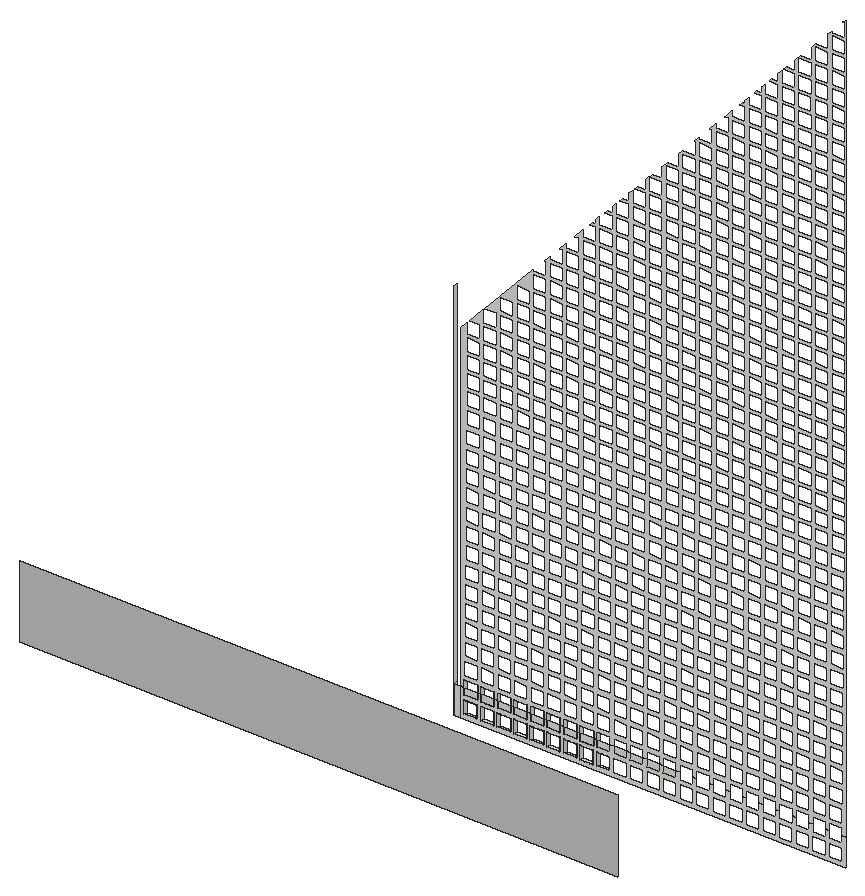
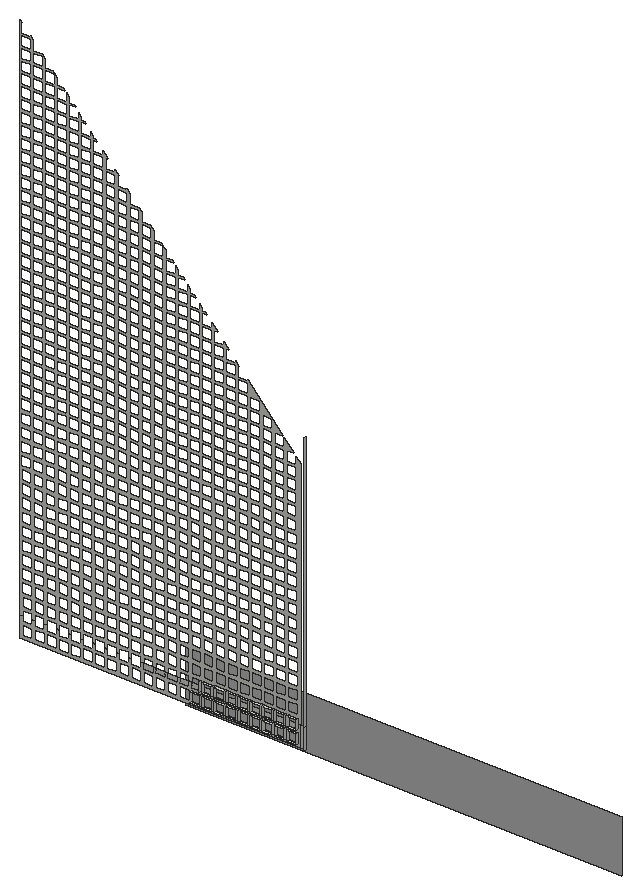
# SketchUp Ruby script. Lengths in inches.
U = 1.inch
M = Sketchup.active_model
def pt(a) = Geom::Point3d.new(a.map { |v| v * U })
def face(e, loops, mat)
  f = e.add_face(loops[0].map { |a| pt(a) })
  loops[1..].each { |l| e.add_face(l.map { |a| pt(a) }).erase! }
  f.material = f.back_material = mat if mat
  f
end
# faces: each face lists its corners as indices into pts; further lists are holes
def faces(e, pts, list, mat = nil) = list.each { |f| face(e, (f[0].is_a?(Array) ? f : [f]).map { |l| l.map { |i| pts[i] } }, mat) }
# xy, xz, yz: faces in a plane at the given z, y or x. An outline is a flat list of corners, or four numbers for a rectangle; further outlines are holes
def ring(l) = l.size == 4 ? [[l[0], l[1]], [l[2], l[1]], [l[2], l[3]], [l[0], l[3]]] : l.each_slice(2).to_a
def flat(e, list, mat, &to3) = list.each { |f| face(e, (f[0].is_a?(Array) ? f : [f]).map { |l| ring(l).map { |u, v| to3.(u, v) } }, mat) }
def xy(e, z, list, mat = nil) = flat(e, list, mat) { |x, y| [x, y, z] }
def xz(e, y, list, mat = nil) = flat(e, list, mat) { |x, z| [x, y, z] }
def yz(e, x, list, mat = nil) = flat(e, list, mat) { |y, z| [x, y, z] }
def lines(e, pts, list) = list.each { |a, b| e.add_line(pt(pts[a]), pt(pts[b])) }
# prism: a flat outline (further loops are holes) pulled along v
def prism(e, loops, v, mat = nil)
  f = face(e, loops, mat); d = Geom::Vector3d.new(v.map { |x| x * U })
  f.pushpull(f.normal.samedirection?(d) ? d.length : -d.length)
end
def box(e, o, s, mat = nil) = prism(e, [[o, [o[0] + s[0], o[1], o[2]], [o[0] + s[0], o[1] + s[1], o[2]], [o[0], o[1] + s[1], o[2]]]], [0, 0, s[2]], mat)
def at(x, y, z, deg = 0) = Geom::Transformation.translation(pt([x, y, z])) * Geom::Transformation.rotation(ORIGIN, Z_AXIS, deg.degrees)
def axes(o, x, y, z) = Geom::Transformation.new([*x, 0, *y, 0, *z, 0, *pt(o).to_a, 1])
def part(name) = M.definitions.add(name)
# library, detail: a bought-in or finely detailed component or shape, given as its bounding box
def library(name, o, s) = part(name).tap { |d| box(d.entities, o, s) }
def detail(e, o, s) = box(e.add_group.entities, o, s)
def put(e, d, t, mat = nil) = e.add_instance(d, t).tap { |i| i.material = mat if mat }
def group(e, t, mat = nil) = e.add_group.tap { |g| g.transformation = t; g.material = mat if mat }.entities
root = M.entities
M.materials.add("[Color M02]").color = [198, 198, 198]
xy(root,259.68,[[432.73,480.14,435.05,480.77],[435.65,480.14,437.96,480.77],[438.56,480.14,440.87,480.77],[441.47,480.14,443.78,480.77],[444.38,480.14,446.69,480.77],
  [447.29,480.14,449.61,480.77],[450.21,480.14,452.52,480.77],[453.12,480.14,455.43,480.77],[456.03,480.14,458.34,480.77]])
xy(root,262,[[432.73,480.14,435.05,480.77],[435.65,480.14,437.96,480.77],[438.56,480.14,440.87,480.77],[441.47,480.14,443.78,480.77],[444.38,480.14,446.69,480.77],
  [447.29,480.14,449.61,480.77],[450.21,480.14,452.52,480.77],[453.12,480.14,455.43,480.77],[456.03,480.14,458.34,480.77]])
xy(root,262.73,[[432.76,480.14,435.08,480.77],[435.68,480.14,437.99,480.77],[438.59,480.14,440.9,480.77],[441.5,480.14,443.8125,480.77],[444.41,480.14,446.72,480.77],
  [447.32,480.14,449.64,480.77],[450.24,480.14,452.55,480.77],[453.15,480.14,455.46,480.77]])
xy(root,265.04,[[432.76,480.14,435.08,480.77],[435.68,480.14,437.99,480.77],[438.59,480.14,440.9,480.77],[441.5,480.14,443.8125,480.77],[444.41,480.14,446.72,480.77],
  [447.32,480.14,449.64,480.77],[450.24,480.14,452.55,480.77],[453.15,480.14,455.46,480.77]])
xz(root,469.875,[[363.02,251.0625,468.02,263.89]],"[Color M02]")
xz(root,480.14,[[430.97,258.95,432.11,263.89],[[432.11,258.95,499.71,258.95,499.71,263.89,499.14,263.89,499.14,262.73,496.83,262.73,496.83,263.89,496.23,263.89,496.23,262.73,493.92,262.73,493.92,263.89,493.32,263.89,493.32,262.73,491,262.73,491,263.89,490.4,263.89,490.4,262.73,488.09,262.73,488.09,263.89,487.49,263.89,487.49,262.73,485.18,262.73,485.18,263.89,484.58,263.89,484.58,262.73,482.27,262.73,482.27,263.89,481.67,263.89,481.67,262.73,479.36,262.73,479.36,263.89,478.76,263.89,478.76,262.73,476.44,262.73,476.44,263.89,475.84,263.89,475.84,262.73,473.53,262.73,473.53,263.89,472.93,263.89,472.93,262.73,470.62,262.73,470.62,263.89,470.02,263.89,470.02,262.73,467.71,262.73,467.71,263.89,467.11,263.89,467.11,262.73,464.8,262.73,464.8,263.89,464.2,263.89,464.2,262.73,461.88,262.73,461.88,263.89,461.28,263.89,461.28,262.73,458.97,262.73,458.97,263.89,458.37,263.89,458.37,262.73,456.06,262.73,456.06,263.89,455.46,263.89,455.46,262.73,453.15,262.73,453.15,263.89,452.55,263.89,452.55,262.73,450.24,262.73,450.24,263.89,449.64,263.89,449.64,262.73,447.32,262.73,447.32,263.89,446.72,263.89,446.72,262.73,444.41,262.73,444.41,263.89,443.8125,263.89,443.8125,262.73,441.5,262.73,441.5,263.89,440.9,263.89,440.9,262.73,438.59,262.73,438.59,263.89,437.99,263.89,437.99,262.73,435.68,262.73,435.68,263.89,435.08,263.89,435.08,262.73,432.76,262.73,432.76,263.89,432.11,263.89],[496.8,259.68,499.11,262],[493.89,259.68,496.2,262],[490.97,259.68,493.29,262],[488.0625,259.68,490.375,262],[485.15,259.68,487.46,262],[482.24,259.68,484.55,262],[479.33,259.68,481.64,262],[476.41,259.68,478.73,262],[473.5,259.68,475.81,262],[470.59,259.68,472.9,262],[467.68,259.68,469.99,262],[464.77,259.68,467.08,262],[461.85,259.68,464.17,262],[458.94,259.68,461.25,262],[456.03,259.68,458.34,262],[453.12,259.68,455.43,262],[450.21,259.68,452.52,262],[447.29,259.68,449.61,262],[444.38,259.68,446.69,262],[441.47,259.68,443.78,262],[438.56,259.68,440.87,262],[435.65,259.68,437.96,262],[432.73,259.68,435.05,262]],[432.76,262.73,435.08,263.89],[435.68,262.73,437.99,263.89],[438.59,262.73,440.9,263.89],
  [441.5,262.73,443.8125,263.89],[444.41,262.73,446.72,263.89],[447.32,262.73,449.64,263.89],[450.24,262.73,452.55,263.89],[453.15,262.73,455.46,263.89],
  [456.06,262.73,458.37,263.89],[458.97,262.73,461.28,263.89],[461.88,262.73,464.2,263.89],[464.8,262.73,467.11,263.89],[467.71,262.73,470.02,263.89],
  [[432.11,263.89,432.76,263.89,432.76,265.04,435.08,265.04,435.08,263.89,435.68,263.89,435.68,265.04,437.99,265.04,437.99,263.89,438.59,263.89,438.59,265.04,440.9,265.04,440.9,263.89,441.5,263.89,441.5,265.04,443.8125,265.04,443.8125,263.89,444.41,263.89,444.41,265.04,446.72,265.04,446.72,263.89,447.32,263.89,447.32,265.04,449.64,265.04,449.64,263.89,450.24,263.89,450.24,265.04,452.55,265.04,452.55,263.89,453.15,263.89,453.15,265.04,455.46,265.04,455.46,263.89,456.06,263.89,456.06,265.04,458.37,265.04,458.37,263.89,458.97,263.89,458.97,265.04,461.28,265.04,461.28,263.89,461.88,263.89,461.88,265.04,464.2,265.04,464.2,263.89,464.8,263.89,464.8,265.04,467.11,265.04,467.11,263.89,467.71,263.89,467.71,265.04,470.02,265.04,470.02,263.89,470.62,263.89,470.62,265.04,472.93,265.04,472.93,263.89,473.53,263.89,473.53,265.04,475.84,265.04,475.84,263.89,476.44,263.89,476.44,265.04,478.76,265.04,478.76,263.89,479.36,263.89,479.36,265.04,481.67,265.04,481.67,263.89,482.27,263.89,482.27,265.04,484.58,265.04,484.58,263.89,485.18,263.89,485.18,265.04,487.49,265.04,487.49,263.89,488.09,263.89,488.09,265.04,490.4,265.04,490.4,263.89,491,263.89,491,265.04,493.32,265.04,493.32,263.89,493.92,263.89,493.92,265.04,496.23,265.04,496.23,263.89,496.83,263.89,496.83,265.04,499.14,265.04,499.14,263.89,499.71,263.89,499.71,392.36,499.28,391.9,499.58,391.9,499.58,389.59,497.26,389.59,497.26,389.75,496.66,389.11,496.66,386.84,494.54,386.84,493.75,386,493.75,384.09,491.96,384.09,491.64,383.75,491.55,383.65,493.75,383.65,493.75,381.34,491.4375,381.34,491.4375,383.53,490.84,382.89,490.84,381.34,489.38,381.34,488.97,380.9,490.84,380.9,490.84,378.59,488.53,378.59,488.53,380.43,487.93,379.79,487.93,378.59,486.8,378.59,486.39,378.15,487.93,378.15,487.93,375.84,485.61,375.84,485.61,377.32,485.02,376.68,485.02,375.84,484.23,375.84,483.82,375.4,485.02,375.4,485.02,373.09,482.7,373.09,482.7,374.21,482.1,373.57,482.1,373.09,481.65,373.09,481.18,372.59,482.1,372.59,482.1,370.27,479.79,370.27,479.79,371.11,479.19,370.47,479.19,370.27,479.01,370.27,478.54,369.77,479.19,369.77,479.19,367.46,476.88,367.46,476.88,368,475.91,366.96,476.28,366.96,476.28,364.65,473.97,364.65,473.97,364.89,473.27,364.15,473.37,364.15,473.37,361.84,471.1,361.84,470.45,361.14,470.45,359.02,468.47,359.02,467.54,358.04,467.54,356.21,465.83,356.21,465.36,355.71,467.54,355.71,467.54,353.4,465.23,353.4,465.23,355.57,464.63,354.93,464.63,353.4,463.19,353.4,462.73,352.9,464.63,352.9,464.63,350.59,462.32,350.59,462.32,352.46,461.72,351.82,461.72,350.59,460.56,350.59,460.09,350.09,461.72,350.09,461.72,347.77,459.41,347.77,459.41,349.36,458.81,348.72,458.81,347.77,457.92,347.77,457.45,347.27,458.81,347.27,458.81,344.96,456.49,344.96,456.49,346.25,455.89,345.61,455.89,344.96,455.29,344.96,454.82,344.46,455.89,344.46,455.89,342.15,453.58,342.15,453.58,343.14,452.18,341.65,452.98,341.65,452.98,339.34,450.67,339.34,450.67,340.04,449.55,338.84,450.07,338.84,450.07,336.52,447.76,336.52,447.76,336.93,446.91,336.02,447.16,336.02,447.16,333.71,444.85,333.71,444.85,333.82,436.37,324.77,438.42,324.77,438.42,322.46,436.11,322.46,436.11,324.5,433.73,321.96,435.51,321.96,435.51,319.65,433.2,319.65,433.2,321.39,432.11,320.24],[497.26,375.84,499.58,378.15],[494.33,373.09,496.64,375.4],[497.26,373.09,499.58,375.4],[494.33,370.27,496.64,372.59],[497.26,370.27,499.58,372.59],[485.59,370.27,487.9,372.59],[488.53,370.27,490.84,372.59],[488.5,373.09,490.8125,375.4],[491.4375,373.09,493.75,375.4],[491.41,375.84,493.73,378.15],[494.35,375.84,496.66,378.15],[494.33,378.59,496.64,380.9],[497.26,378.59,499.58,380.9],[494.33,381.34,496.64,383.65],[497.26,381.34,499.58,383.65],[465.23,350.59,467.54,352.9],[462.32,347.77,464.63,350.09],[465.23,347.77,467.54,350.09],[459.41,344.96,461.72,347.27],[462.32,344.96,464.63,347.27],[465.23,344.96,467.54,347.27],[468.14,344.96,470.45,347.27],[471.05,344.96,473.37,347.27],[473.97,344.96,476.28,347.27],[476.88,344.96,479.19,347.27],[479.79,344.96,482.1,347.27],[482.7,344.96,485.02,347.27],[485.61,344.96,487.93,347.27],[488.53,344.96,490.84,347.27],[491.4375,344.96,493.75,347.27],[494.35,344.96,496.66,347.27],[497.26,344.96,499.58,347.27],[468.14,347.77,470.45,350.09],[471.05,347.77,473.37,350.09],[473.97,347.77,476.28,350.09],[476.88,347.77,479.19,350.09],[479.79,347.77,482.1,350.09],[482.7,347.77,485.02,350.09],[485.61,347.77,487.93,350.09],[488.53,347.77,490.84,350.09],[491.4375,347.77,493.75,350.09],[494.35,347.77,496.66,350.09],[497.26,347.77,499.58,350.09],[468.14,350.59,470.45,352.9],[471.05,350.59,473.37,352.9],[473.97,350.59,476.28,352.9],[476.88,350.59,479.19,352.9],[479.79,350.59,482.1,352.9],[482.7,350.59,485.02,352.9],[485.61,350.59,487.93,352.9],[488.53,350.59,490.84,352.9],[491.4375,350.59,493.75,352.9],[494.35,350.59,496.66,352.9],[497.26,350.59,499.58,352.9],[468.14,353.4,470.45,355.71],[471.05,353.4,473.37,355.71],[473.97,353.4,476.28,355.71],[476.88,353.4,479.19,355.71],[479.79,353.4,482.1,355.71],[482.7,353.4,485.02,355.71],[485.61,353.4,487.93,355.71],[488.53,353.4,490.84,355.71],[491.4375,353.4,493.75,355.71],[494.35,353.4,496.66,355.71],[497.26,353.4,499.58,355.71],[479.79,367.46,482.1,369.77],[482.7,367.46,485.02,369.77],[491.4375,367.46,493.75,369.77],[497.26,367.46,499.58,369.77],[488.53,367.46,490.84,369.77],[485.61,367.46,487.93,369.77],[494.35,367.46,496.66,369.77],[479.79,364.65,482.1,366.96],[485.61,364.65,487.93,366.96],[494.35,364.65,496.66,366.96],[491.4375,364.65,493.75,366.96],[482.7,364.65,485.02,366.96],[488.53,364.65,490.84,366.96],[497.26,364.65,499.58,366.96],[476.88,364.65,479.19,366.96],[488.53,361.84,490.84,364.15],[494.35,361.84,496.66,364.15],[482.7,361.84,485.02,364.15],[485.61,361.84,487.93,364.15],[497.26,361.84,499.58,364.15],[476.88,361.84,479.19,364.15],[473.97,361.84,476.28,364.15],[479.79,361.84,482.1,364.15],[491.4375,361.84,493.75,364.15],[488.53,359.02,490.84,361.34],[494.35,359.02,496.66,361.34],[482.7,359.02,485.02,361.34],[471.05,359.02,473.37,361.34],[497.26,359.02,499.58,361.34],[485.61,359.02,487.93,361.34],[476.88,359.02,479.19,361.34],[473.97,359.02,476.28,361.34],[491.4375,359.02,493.75,361.34],[479.79,359.02,482.1,361.34],[491.4375,356.21,493.75,358.52],[479.79,356.21,482.1,358.52],[473.97,356.21,476.28,358.52],[485.61,356.21,487.93,358.52],[497.26,356.21,499.58,358.52],[468.14,356.21,470.45,358.52],[476.88,356.21,479.19,358.52],[471.05,356.21,473.37,358.52],[482.7,356.21,485.02,358.52],[494.35,356.21,496.66,358.52],[488.53,356.21,490.84,358.52],[456.49,342.15,458.81,344.46],[459.41,342.15,461.72,344.46],[462.32,342.15,464.63,344.46],[465.23,342.15,467.54,344.46],[468.14,342.15,470.45,344.46],[471.05,342.15,473.37,344.46],[473.97,342.15,476.28,344.46],[476.88,342.15,479.19,344.46],[479.79,342.15,482.1,344.46],[482.7,342.15,485.02,344.46],[485.61,342.15,487.93,344.46],[488.53,342.15,490.84,344.46],[491.4375,342.15,493.75,344.46],[494.35,342.15,496.66,344.46],[497.26,342.15,499.58,344.46],[453.58,339.34,455.89,341.65],[456.49,339.34,458.81,341.65],[459.41,339.34,461.72,341.65],[462.32,339.34,464.63,341.65],[465.23,339.34,467.54,341.65],[468.14,339.34,470.45,341.65],[471.05,339.34,473.37,341.65],[473.97,339.34,476.28,341.65],[476.88,339.34,479.19,341.65],[479.79,339.34,482.1,341.65],[482.7,339.34,485.02,341.65],[485.61,339.34,487.93,341.65],[488.53,339.34,490.84,341.65],[491.4375,339.34,493.75,341.65],[494.35,339.34,496.66,341.65],[497.26,339.34,499.58,341.65],[450.67,336.52,452.98,338.84],[453.58,336.52,455.89,338.84],[456.49,336.52,458.81,338.84],[459.41,336.52,461.72,338.84],[462.32,336.52,464.63,338.84],[465.23,336.52,467.54,338.84],[468.14,336.52,470.45,338.84],[471.05,336.52,473.37,338.84],[473.97,336.52,476.28,338.84],[476.88,336.52,479.19,338.84],[479.79,336.52,482.1,338.84],[482.7,336.52,485.02,338.84],[485.61,336.52,487.93,338.84],[488.53,336.52,490.84,338.84],[491.4375,336.52,493.75,338.84],[494.35,336.52,496.66,338.84],[497.26,336.52,499.58,338.84],[447.76,333.71,450.07,336.02],[450.67,333.71,452.98,336.02],[453.58,333.71,455.89,336.02],[456.49,333.71,458.81,336.02],[459.41,333.71,461.72,336.02],[462.32,333.71,464.63,336.02],[465.23,333.71,467.54,336.02],[468.14,333.71,470.45,336.02],[471.05,333.71,473.37,336.02],[473.97,333.71,476.28,336.02],[476.88,333.71,479.19,336.02],[479.79,333.71,482.1,336.02],[482.7,333.71,485.02,336.02],[485.61,333.71,487.93,336.02],[488.53,333.71,490.84,336.02],[491.4375,333.71,493.75,336.02],[494.35,333.71,496.66,336.02],[497.26,333.71,499.58,336.02],[444.85,330.9,447.16,333.21],[447.76,330.9,450.07,333.21],[450.67,330.9,452.98,333.21],[453.58,330.9,455.89,333.21],[456.49,330.9,458.81,333.21],[459.41,330.9,461.72,333.21],[462.32,330.9,464.63,333.21],[465.23,330.9,467.54,333.21],[468.14,330.9,470.45,333.21],[471.05,330.9,473.37,333.21],[473.97,330.9,476.28,333.21],[476.88,330.9,479.19,333.21],[479.79,330.9,482.1,333.21],[482.7,330.9,485.02,333.21],[485.61,330.9,487.93,333.21],[488.53,330.9,490.84,333.21],[491.4375,330.9,493.75,333.21],[494.35,330.9,496.66,333.21],[497.26,330.9,499.58,333.21],[441.93,328.09,444.25,330.4],[444.85,328.09,447.16,330.4],[447.76,328.09,450.07,330.4],[450.67,328.09,452.98,330.4],[453.58,328.09,455.89,330.4],[456.49,328.09,458.81,330.4],[459.41,328.09,461.72,330.4],[462.32,328.09,464.63,330.4],[465.23,328.09,467.54,330.4],[468.14,328.09,470.45,330.4],[471.05,328.09,473.37,330.4],[473.97,328.09,476.28,330.4],[476.88,328.09,479.19,330.4],[479.79,328.09,482.1,330.4],[482.7,328.09,485.02,330.4],[485.61,328.09,487.93,330.4],[488.53,328.09,490.84,330.4],[491.4375,328.09,493.75,330.4],[494.35,328.09,496.66,330.4],[497.26,328.09,499.58,330.4],[439.02,325.27,441.33,327.59],[441.93,325.27,444.25,327.59],[444.85,325.27,447.16,327.59],[447.76,325.27,450.07,327.59],[450.67,325.27,452.98,327.59],[453.58,325.27,455.89,327.59],[456.49,325.27,458.81,327.59],[459.41,325.27,461.72,327.59],[462.32,325.27,464.63,327.59],[465.23,325.27,467.54,327.59],[468.14,325.27,470.45,327.59],[471.05,325.27,473.37,327.59],[473.97,325.27,476.28,327.59],[476.88,325.27,479.19,327.59],[479.79,325.27,482.1,327.59],[482.7,325.27,485.02,327.59],[485.61,325.27,487.93,327.59],[488.53,325.27,490.84,327.59],[491.4375,325.27,493.75,327.59],[494.35,325.27,496.66,327.59],[497.26,325.27,499.58,327.59],[439.02,322.46,441.33,324.77],[441.93,322.46,444.25,324.77],[444.85,322.46,447.16,324.77],[447.76,322.46,450.07,324.77],[450.67,322.46,452.98,324.77],[453.58,322.46,455.89,324.77],[456.49,322.46,458.81,324.77],[459.41,322.46,461.72,324.77],[462.32,322.46,464.63,324.77],[465.23,322.46,467.54,324.77],[468.14,322.46,470.45,324.77],[471.05,322.46,473.37,324.77],[473.97,322.46,476.28,324.77],[476.88,322.46,479.19,324.77],[479.79,322.46,482.1,324.77],[482.7,322.46,485.02,324.77],[485.61,322.46,487.93,324.77],[488.53,322.46,490.84,324.77],[491.4375,322.46,493.75,324.77],[494.35,322.46,496.66,324.77],[497.26,322.46,499.58,324.77],[436.11,319.65,438.42,321.96],[439.02,319.65,441.33,321.96],[441.93,319.65,444.25,321.96],[444.85,319.65,447.16,321.96],[447.76,319.65,450.07,321.96],[450.67,319.65,452.98,321.96],[453.58,319.65,455.89,321.96],[456.49,319.65,458.81,321.96],[459.41,319.65,461.72,321.96],[462.32,319.65,464.63,321.96],[465.23,319.65,467.54,321.96],[468.14,319.65,470.45,321.96],[471.05,319.65,473.37,321.96],[473.97,319.65,476.28,321.96],[476.88,319.65,479.19,321.96],[479.79,319.65,482.1,321.96],[482.7,319.65,485.02,321.96],[485.61,319.65,487.93,321.96],[488.53,319.65,490.84,321.96],[491.4375,319.65,493.75,321.96],[494.35,319.65,496.66,321.96],[497.26,319.65,499.58,321.96],[433.2,316.84,435.51,319.15],[436.11,316.84,438.42,319.15],[439.02,316.84,441.33,319.15],[441.93,316.84,444.25,319.15],[444.85,316.84,447.16,319.15],[447.76,316.84,450.07,319.15],[450.67,316.84,452.98,319.15],[453.58,316.84,455.89,319.15],[456.49,316.84,458.81,319.15],[459.41,316.84,461.72,319.15],[462.32,316.84,464.63,319.15],[465.23,316.84,467.54,319.15],[468.14,316.84,470.45,319.15],[471.05,316.84,473.37,319.15],[473.97,316.84,476.28,319.15],[476.88,316.84,479.19,319.15],[479.79,316.84,482.1,319.15],[482.7,316.84,485.02,319.15],[485.61,316.84,487.93,319.15],[488.53,316.84,490.84,319.15],[491.4375,316.84,493.75,319.15],[494.35,316.84,496.66,319.15],[497.26,316.84,499.58,319.15],[433.2,314.02,435.51,316.34],[436.11,314.02,438.42,316.34],[439.02,314.02,441.33,316.34],[441.93,314.02,444.25,316.34],[444.85,314.02,447.16,316.34],[447.76,314.02,450.07,316.34],[450.67,314.02,452.98,316.34],[453.58,314.02,455.89,316.34],[456.49,314.02,458.81,316.34],[459.41,314.02,461.72,316.34],[462.32,314.02,464.63,316.34],[465.23,314.02,467.54,316.34],[468.14,314.02,470.45,316.34],[471.05,314.02,473.37,316.34],[473.97,314.02,476.28,316.34],[476.88,314.02,479.19,316.34],[479.79,314.02,482.1,316.34],[482.7,314.02,485.02,316.34],[485.61,314.02,487.93,316.34],[488.53,314.02,490.84,316.34],[491.4375,314.02,493.75,316.34],[494.35,314.02,496.66,316.34],[497.26,314.02,499.58,316.34],[450.67,311.21,452.98,313.52],[453.58,311.21,455.89,313.52],[439.02,311.21,441.33,313.52],[433.2,311.21,435.51,313.52],[494.35,311.21,496.66,313.52],[476.88,311.21,479.19,313.52],[465.23,311.21,467.54,313.52],[441.93,311.21,444.25,313.52],[471.05,311.21,473.37,313.52],[468.14,311.21,470.45,313.52],[444.85,311.21,447.16,313.52],[482.7,311.21,485.02,313.52],[456.49,311.21,458.81,313.52],[491.4375,311.21,493.75,313.52],[485.61,311.21,487.93,313.52],[436.11,311.21,438.42,313.52],[479.79,311.21,482.1,313.52],[488.53,311.21,490.84,313.52],[462.32,311.21,464.63,313.52],[497.26,311.21,499.58,313.52],[447.76,311.21,450.07,313.52],[459.41,311.21,461.72,313.52],[473.97,311.21,476.28,313.52],[433.2,308.4,435.51,310.71],[436.11,308.4,438.42,310.71],[439.02,308.4,441.33,310.71],[441.93,308.4,444.25,310.71],[444.85,308.4,447.16,310.71],[447.76,308.4,450.07,310.71],[450.67,308.4,452.98,310.71],[453.58,308.4,455.89,310.71],[456.49,308.4,458.81,310.71],[459.41,308.4,461.72,310.71],[462.32,308.4,464.63,310.71],[465.23,308.4,467.54,310.71],[468.14,308.4,470.45,310.71],[471.05,308.4,473.37,310.71],[473.97,308.4,476.28,310.71],[476.88,308.4,479.19,310.71],[479.79,308.4,482.1,310.71],[482.7,308.4,485.02,310.71],[485.61,308.4,487.93,310.71],[488.53,308.4,490.84,310.71],[491.4375,308.4,493.75,310.71],[494.35,308.4,496.66,310.71],[497.26,308.4,499.58,310.71],[433.17,305.35,435.48,307.67],[436.08,305.35,438.39,307.67],[438.99,305.35,441.31,307.67],[441.91,305.35,444.22,307.67],[444.82,305.35,447.13,307.67],[447.73,305.35,450.04,307.67],[450.64,305.35,452.95,307.67],[453.55,305.35,455.87,307.67],[456.47,305.35,458.78,307.67],[459.38,305.35,461.69,307.67],[462.29,305.35,464.6,307.67],[465.2,305.35,467.51,307.67],[468.11,305.35,470.43,307.67],[471.03,305.35,473.34,307.67],[473.9375,305.35,476.25,307.67],[476.85,305.35,479.16,307.67],[479.76,305.35,482.07,307.67],[482.67,305.35,484.99,307.67],[485.59,305.35,487.9,307.67],[488.5,305.35,490.81,307.67],[491.41,305.35,493.72,307.67],[494.32,305.35,496.63,307.67],[497.23,305.35,499.55,307.67],[433.14,302.31,435.45,304.62],[436.05,302.31,438.36,304.62],[438.96,302.31,441.28,304.62],[441.875,302.31,444.1875,304.62],[444.79,302.31,447.1,304.62],[447.7,302.31,450.01,304.62],[450.61,302.31,452.92,304.62],[453.52,302.31,455.84,304.62],[456.4375,302.31,458.75,304.62],[459.35,302.31,461.66,304.62],[462.26,302.31,464.57,304.62],[465.17,302.31,467.48,304.62],[468.08,302.31,470.4,304.62],[471,302.31,473.31,304.62],[473.91,302.31,476.22,304.62],[476.82,302.31,479.13,304.62],[479.73,302.31,482.04,304.62],[482.64,302.31,484.96,304.62],[485.56,302.31,487.87,304.62],[488.47,302.31,490.78,304.62],[491.38,302.31,493.69,304.62],[494.29,302.31,496.61,304.62],[497.2,302.31,499.52,304.62],[433.11,299.27,435.42,301.58],[436.02,299.27,438.34,301.58],[438.93,299.27,441.25,301.58],[441.85,299.27,444.16,301.58],[444.76,299.27,447.07,301.58],[447.67,299.27,449.98,301.58],[450.58,299.27,452.9,301.58],[453.5,299.27,455.81,301.58],[456.41,299.27,458.72,301.58],[459.32,299.27,461.63,301.58],[462.23,299.27,464.54,301.58],[465.14,299.27,467.46,301.58],[468.06,299.27,470.37,301.58],[470.97,299.27,473.28,301.58],[473.88,299.27,476.19,301.58],[476.79,299.27,479.1,301.58],[479.7,299.27,482.02,301.58],[482.62,299.27,484.93,301.58],[485.53,299.27,487.84,301.58],[488.44,299.27,490.75,301.58],[491.35,299.27,493.66,301.58],[494.26,299.27,496.58,301.58],[497.18,299.27,499.49,301.58],[433.08,296.22,435.39,298.53],[435.99,296.22,438.31,298.53],[438.91,296.22,441.22,298.53],[441.82,296.22,444.13,298.53],[444.73,296.22,447.04,298.53],[447.64,296.22,449.95,298.53],[450.55,296.22,452.87,298.53],[453.47,296.22,455.78,298.53],[456.38,296.22,458.69,298.53],[459.29,296.22,461.6,298.53],[462.2,296.22,464.51,298.53],[465.11,296.22,467.43,298.53],[468.03,296.22,470.34,298.53],[470.9375,296.22,473.25,298.53],[473.85,296.22,476.16,298.53],[476.76,296.22,479.07,298.53],[479.67,296.22,481.99,298.53],[482.59,296.22,484.9,298.53],[485.5,296.22,487.8125,298.53],[488.41,296.22,490.72,298.53],[491.32,296.22,493.64,298.53],[494.23,296.22,496.55,298.53],[497.15,296.22,499.46,298.53],[433.05,293.18,435.37,295.49],[435.96,293.18,438.28,295.49],[438.875,293.18,441.1875,295.49],[441.79,293.18,444.1,295.49],[444.7,293.18,447.01,295.49],[447.61,293.18,449.93,295.49],[450.53,293.18,452.84,295.49],[453.4375,293.18,455.75,295.49],[456.35,293.18,458.66,295.49],[459.26,293.18,461.57,295.49],[462.17,293.18,464.49,295.49],[465.09,293.18,467.4,295.49],[468,293.18,470.31,295.49],[470.91,293.18,473.22,295.49],[473.82,293.18,476.13,295.49],[476.73,293.18,479.05,295.49],[479.65,293.18,481.96,295.49],[482.56,293.18,484.87,295.49],[485.47,293.18,487.78,295.49],[488.38,293.18,490.69,295.49],[491.29,293.18,493.61,295.49],[494.21,293.18,496.52,295.49],[497.12,293.18,499.43,295.49],[433.02,290.13,435.34,292.44],[435.9375,290.13,438.25,292.44],[438.85,290.13,441.16,292.44],[441.76,290.13,444.07,292.44],[444.67,290.13,446.98,292.44],[447.58,290.13,449.9,292.44],[450.5,290.13,452.81,292.44],[453.41,290.13,455.72,292.44],[456.32,290.13,458.63,292.44],[459.23,290.13,461.54,292.44],[462.14,290.13,464.46,292.44],[465.06,290.13,467.37,292.44],[467.97,290.13,470.28,292.44],[470.88,290.13,473.19,292.44],[473.79,290.13,476.1,292.44],[476.7,290.13,479.02,292.44],[479.62,290.13,481.93,292.44],[482.53,290.13,484.84,292.44],[485.44,290.13,487.75,292.44],[488.35,290.13,490.67,292.44],[491.26,290.13,493.58,292.44],[494.18,290.13,496.49,292.44],[497.09,290.13,499.4,292.44],[432.99,287.09,435.31,289.4],[435.91,287.09,438.22,289.4],[438.82,287.09,441.13,289.4],[441.73,287.09,444.04,289.4],[444.64,287.09,446.96,289.4],[447.56,287.09,449.87,289.4],[450.47,287.09,452.78,289.4],[453.38,287.09,455.69,289.4],[456.29,287.09,458.6,289.4],[459.2,287.09,461.52,289.4],[462.12,287.09,464.43,289.4],[465.03,287.09,467.34,289.4],[467.9375,287.09,470.25,289.4],[470.85,287.09,473.16,289.4],[473.76,287.09,476.08,289.4],[476.68,287.09,478.99,289.4],[479.59,287.09,481.9,289.4],[482.5,287.09,484.8125,289.4],[485.41,287.09,487.72,289.4],[488.32,287.09,490.64,289.4],[491.24,287.09,493.55,289.4],[494.15,287.09,496.46,289.4],[497.06,287.09,499.37,289.4],[432.97,284.04,435.28,286.35],[435.88,284.04,438.19,286.35],[438.79,284.04,441.1,286.35],[441.7,284.04,444.01,286.35],[444.61,284.04,446.93,286.35],[447.53,284.04,449.84,286.35],[450.4375,284.04,452.75,286.35],[453.35,284.04,455.66,286.35],[456.26,284.04,458.57,286.35],[459.17,284.04,461.49,286.35],[462.09,284.04,464.4,286.35],[465,284.04,467.3125,286.35],[467.91,284.04,470.22,286.35],[470.82,284.04,473.13,286.35],[473.73,284.04,476.05,286.35],[476.65,284.04,478.96,286.35],[479.56,284.04,481.87,286.35],[482.47,284.04,484.78,286.35],[485.38,284.04,487.7,286.35],[488.29,284.04,490.61,286.35],[491.21,284.04,493.52,286.35],[494.12,284.04,496.43,286.35],[497.03,284.04,499.34,286.35],[432.9375,281,435.25,283.31],[435.85,281,438.16,283.31],[438.76,281,441.07,283.31],[441.67,281,443.99,283.31],[444.59,281,446.9,283.31],[447.5,281,449.81,283.31],[450.41,281,452.72,283.31],[453.32,281,455.63,283.31],[456.23,281,458.55,283.31],[459.15,281,461.46,283.31],[462.06,281,464.37,283.31],[464.97,281,467.28,283.31],[467.88,281,470.19,283.31],[470.79,281,473.11,283.31],[473.71,281,476.02,283.31],[476.62,281,478.93,283.31],[479.53,281,481.84,283.31],[482.44,281,484.75,283.31],[485.35,281,487.67,283.31],[488.27,281,490.58,283.31],[491.18,281,493.49,283.31],[494.09,281,496.4,283.31],[497,281,499.3125,283.31],[432.91,277.95,435.22,280.26],[435.82,277.95,438.13,280.26],[438.73,277.95,441.04,280.26],[441.64,277.95,443.96,280.26],[444.56,277.95,446.87,280.26],[447.47,277.95,449.78,280.26],[450.38,277.95,452.69,280.26],[453.29,277.95,455.6,280.26],[456.2,277.95,458.52,280.26],[459.12,277.95,461.43,280.26],[462.03,277.95,464.34,280.26],[464.94,277.95,467.25,280.26],[467.85,277.95,470.16,280.26],[470.76,277.95,473.08,280.26],[473.68,277.95,475.99,280.26],[476.59,277.95,478.9,280.26],[479.5,277.95,481.8125,280.26],[482.41,277.95,484.73,280.26],[485.32,277.95,487.64,280.26],[488.24,277.95,490.55,280.26],[491.15,277.95,493.46,280.26],[494.0625,277.95,496.375,280.26],[496.97,277.95,499.29,280.26],[432.88,274.91,435.19,277.22],[435.79,274.91,438.1,277.22],[438.7,274.91,441.02,277.22],[441.62,274.91,443.93,277.22],[444.53,274.91,446.84,277.22],[447.4375,274.91,449.75,277.22],[450.35,274.91,452.66,277.22],[453.26,274.91,455.58,277.22],[456.18,274.91,458.49,277.22],[459.09,274.91,461.4,277.22],[462,274.91,464.3125,277.22],[464.91,274.91,467.22,277.22],[467.82,274.91,470.14,277.22],[470.74,274.91,473.05,277.22],[473.65,274.91,475.96,277.22],[476.56,274.91,478.87,277.22],[479.47,274.91,481.78,277.22],[482.38,274.91,484.7,277.22],[485.3,274.91,487.61,277.22],[488.21,274.91,490.52,277.22],[491.12,274.91,493.43,277.22],[494.03,274.91,496.34,277.22],[496.94,274.91,499.26,277.22],[432.85,271.86,435.16,274.17],[435.76,271.86,438.07,274.17],[438.67,271.86,440.99,274.17],[441.59,271.86,443.9,274.17],[444.5,271.86,446.8125,274.17],[447.41,271.86,449.72,274.17],[450.32,271.86,452.63,274.17],[453.23,271.86,455.55,274.17],[456.15,271.86,458.46,274.17],[459.06,271.86,461.37,274.17],[461.97,271.86,464.28,274.17],[464.88,271.86,467.19,274.17],[467.79,271.86,470.11,274.17],[470.71,271.86,473.02,274.17],[473.62,271.86,475.93,274.17],[476.53,271.86,478.84,274.17],[479.44,271.86,481.76,274.17],[482.35,271.86,484.67,274.17],[485.27,271.86,487.58,274.17],[488.18,271.86,490.49,274.17],[491.09,271.86,493.4,274.17],[494,271.86,496.32,274.17],[496.91,271.86,499.23,274.17],[432.82,268.82,435.13,271.13],[435.73,268.82,438.05,271.13],[438.65,268.82,440.96,271.13],[441.56,268.82,443.87,271.13],[444.47,268.82,446.78,271.13],[447.38,268.82,449.69,271.13],[450.29,268.82,452.61,271.13],[453.21,268.82,455.52,271.13],[456.12,268.82,458.43,271.13],[459.03,268.82,461.34,271.13],[461.94,268.82,464.25,271.13],[464.85,268.82,467.17,271.13],[467.77,268.82,470.08,271.13],[470.68,268.82,472.99,271.13],[473.59,268.82,475.9,271.13],[476.5,268.82,478.8125,271.13],[479.41,268.82,481.73,271.13],[482.33,268.82,484.64,271.13],[485.24,268.82,487.55,271.13],[488.15,268.82,490.46,271.13],[491.0625,268.82,493.375,271.13],[493.97,268.82,496.29,271.13],[496.89,268.82,499.2,271.13],[432.79,265.77,435.1,268.09],[435.7,265.77,438.02,268.09],[438.62,265.77,440.93,268.09],[441.53,265.77,443.84,268.09],[444.44,265.77,446.75,268.09],[447.35,265.77,449.66,268.09],[450.26,265.77,452.58,268.09],[453.18,265.77,455.49,268.09],[456.09,265.77,458.4,268.09],[459,265.77,461.3125,268.09],[461.91,265.77,464.22,268.09],[464.82,265.77,467.14,268.09],[467.74,265.77,470.05,268.09],[470.65,265.77,472.96,268.09],[473.56,265.77,475.87,268.09],[476.47,265.77,478.79,268.09],[479.38,265.77,481.7,268.09],[482.3,265.77,484.61,268.09],[485.21,265.77,487.52,268.09],[488.12,265.77,490.43,268.09],[491.03,265.77,493.35,268.09],[493.94,265.77,496.26,268.09],[496.86,265.77,499.17,268.09],[497.26,384.09,499.58,386.4],[494.35,384.09,496.66,386.4],[497.26,386.84,499.58,389.15],[491.4375,370.27,491.4375,372.47,491.55,372.59,493.75,372.59,493.75,370.27],[482.7,370.27,482.7,372.47,482.8125,372.59,485.02,372.59,485.02,370.27],[485.61,373.09,485.61,375.28,485.72,375.4,487.93,375.4,487.93,373.09],[488.53,375.84,488.53,378.03,488.64,378.15,490.84,378.15,490.84,375.84],[491.4375,378.59,491.4375,380.78,491.55,380.9,493.75,380.9,493.75,378.59]]])
yz(root,430.97,[[480.14,258.95,480.77,263.89],[480.14,263.89,480.77,326.5]])
yz(root,432.73,[[480.14,259.68,480.77,262]])
yz(root,432.76,[[480.14,262.73,480.77,265.04]])
yz(root,435.05,[[480.14,259.68,480.77,262]])
yz(root,435.08,[[480.14,262.73,480.77,265.04]])
yz(root,435.65,[[480.14,259.68,480.77,262]])
yz(root,435.68,[[480.14,262.73,480.77,265.04]])
yz(root,437.96,[[480.14,259.68,480.77,262]])
yz(root,437.99,[[480.14,262.73,480.77,265.04]])
yz(root,438.56,[[480.14,259.68,480.77,262]])
yz(root,438.59,[[480.14,262.73,480.77,265.04]])
yz(root,440.87,[[480.14,259.68,480.77,262]])
yz(root,440.9,[[480.14,262.73,480.77,265.04]])
yz(root,441.47,[[480.14,259.68,480.77,262]])
yz(root,441.5,[[480.14,262.73,480.77,265.04]])
yz(root,443.78,[[480.14,259.68,480.77,262]])
yz(root,443.8125,[[480.14,262.73,480.77,265.04]])
yz(root,444.38,[[480.14,259.68,480.77,262]])
yz(root,444.41,[[480.14,262.73,480.77,265.04]])
yz(root,446.69,[[480.14,259.68,480.77,262]])
yz(root,446.72,[[480.14,262.73,480.77,265.04]])
yz(root,447.29,[[480.14,259.68,480.77,262]])
yz(root,447.32,[[480.14,262.73,480.77,265.04]])
yz(root,449.61,[[480.14,259.68,480.77,262]])
yz(root,449.64,[[480.14,262.73,480.77,265.04]])
yz(root,450.21,[[480.14,259.68,480.77,262]])
yz(root,450.24,[[480.14,262.73,480.77,265.04]])
yz(root,452.52,[[480.14,259.68,480.77,262]])
yz(root,452.55,[[480.14,262.73,480.77,265.04]])
yz(root,453.12,[[480.14,259.68,480.77,262]])
yz(root,453.15,[[480.14,262.73,480.77,265.04]])
yz(root,455.43,[[480.14,259.68,480.77,262]])
yz(root,455.46,[[480.14,262.73,480.77,265.04]])
yz(root,456.03,[[480.14,259.68,480.77,262]])
yz(root,456.06,[[480.14,262.73,480.77,265.04]])
